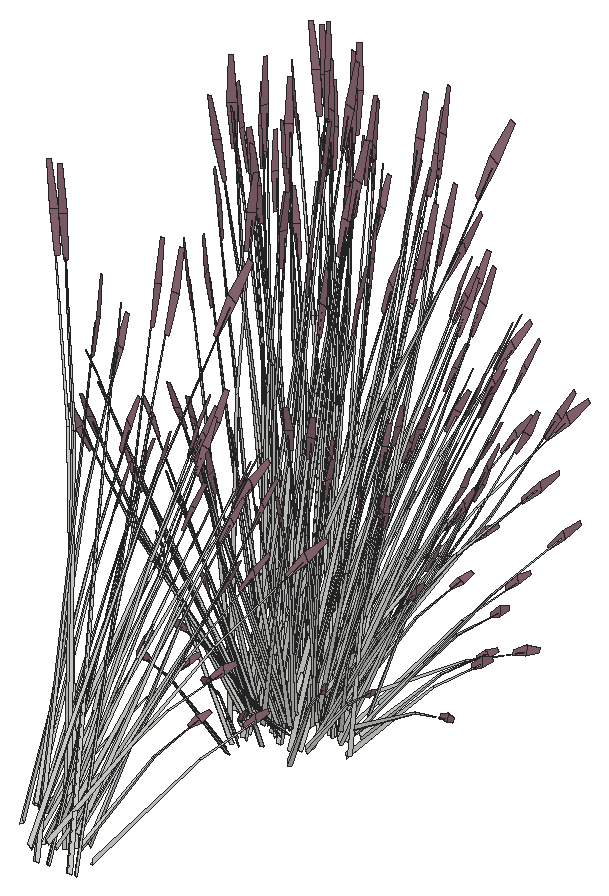
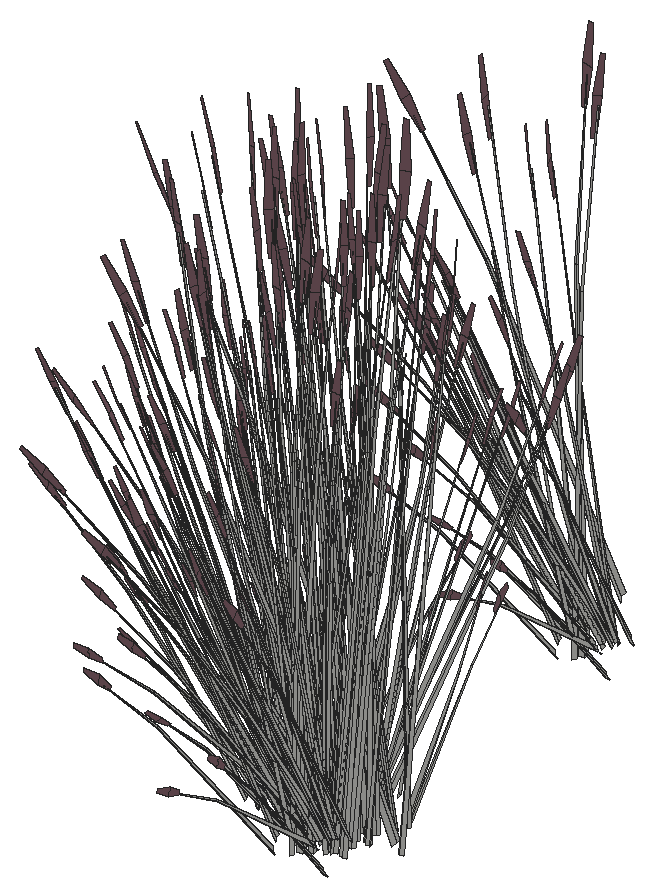
# SketchUp Ruby script. Lengths in inches.
U = 1.inch
M = Sketchup.active_model
def pt(a) = Geom::Point3d.new(a.map { |v| v * U })
def face(e, loops, mat)
  f = e.add_face(loops[0].map { |a| pt(a) })
  loops[1..].each { |l| e.add_face(l.map { |a| pt(a) }).erase! }
  f.material = f.back_material = mat if mat
  f
end
# faces: each face lists its corners as indices into pts; further lists are holes
def faces(e, pts, list, mat = nil) = list.each { |f| face(e, (f[0].is_a?(Array) ? f : [f]).map { |l| l.map { |i| pts[i] } }, mat) }
# xy, xz, yz: faces in a plane at the given z, y or x. An outline is a flat list of corners, or four numbers for a rectangle; further outlines are holes
def ring(l) = l.size == 4 ? [[l[0], l[1]], [l[2], l[1]], [l[2], l[3]], [l[0], l[3]]] : l.each_slice(2).to_a
def flat(e, list, mat, &to3) = list.each { |f| face(e, (f[0].is_a?(Array) ? f : [f]).map { |l| ring(l).map { |u, v| to3.(u, v) } }, mat) }
def xy(e, z, list, mat = nil) = flat(e, list, mat) { |x, y| [x, y, z] }
def xz(e, y, list, mat = nil) = flat(e, list, mat) { |x, z| [x, y, z] }
def yz(e, x, list, mat = nil) = flat(e, list, mat) { |y, z| [x, y, z] }
def lines(e, pts, list) = list.each { |a, b| e.add_line(pt(pts[a]), pt(pts[b])) }
# prism: a flat outline (further loops are holes) pulled along v
def prism(e, loops, v, mat = nil)
  f = face(e, loops, mat); d = Geom::Vector3d.new(v.map { |x| x * U })
  f.pushpull(f.normal.samedirection?(d) ? d.length : -d.length)
end
def box(e, o, s, mat = nil) = prism(e, [[o, [o[0] + s[0], o[1], o[2]], [o[0] + s[0], o[1] + s[1], o[2]], [o[0], o[1] + s[1], o[2]]]], [0, 0, s[2]], mat)
def at(x, y, z, deg = 0) = Geom::Transformation.translation(pt([x, y, z])) * Geom::Transformation.rotation(ORIGIN, Z_AXIS, deg.degrees)
def axes(o, x, y, z) = Geom::Transformation.new([*x, 0, *y, 0, *z, 0, *pt(o).to_a, 1])
def part(name) = M.definitions.add(name)
# library, detail: a bought-in or finely detailed component or shape, given as its bounding box
def library(name, o, s) = part(name).tap { |d| box(d.entities, o, s) }
def detail(e, o, s) = box(e.add_group.entities, o, s)
def put(e, d, t, mat = nil) = e.add_instance(d, t).tap { |i| i.material = mat if mat }
def group(e, t, mat = nil) = e.add_group.tap { |g| g.transformation = t; g.material = mat if mat }.entities
root = M.entities
M.materials.add("LightPink_Translucent").color = [144, 107, 117]
c1 = part("blade")
p = [[2.15,0.21,22],[0,0.17,0],[0.09,0.45,0],[2.18,0.31,22],[2.29,0.31,22],[0.38,0.45,0],
  [2.48,0.24,33],[2.49,0.24,33],[2.48,0.22,33]]
faces(c1.entities,p,[[0,1,2,3],[4,5,2,3],[6,3,4,7],[8,0,3,6]])
c2 = part("seeds")
p = [[0.3,-0.1,1.38],[-0.01,-0.03,1.59],[-0.01,-0.03,0.03],[0.14,-0.07,-0.07],[0.29,-0.03,3],[0.15,0.01,3.11]]
faces(c2.entities,p,[[0,1,2,3],[1,0,4,5]],"LightPink_Translucent")
c3 = part("blade with seeds")
put(c3.entities,c1,at(0,0,0))
put(c3.entities,c2,axes([2.4,0.25,30.99],[1.5799,-0.05474,1.17369],[-0.12525,1.92788,0.29478],[-0.07173,-0.02425,1.56792]))
put(root,c3,axes([76.63,462.61,35.41],[-1.19922,0.48218,-0.1216],[-0.58932,-0.85579,-0.67495],[-0.15822,-0.36063,1.02557]))
put(root,c3,axes([75.6,462.65,35.06],[-1.20468,-0.25962,-0.51099],[0.41292,-0.89013,-0.3958],[-0.11046,-0.35838,0.97773]))
put(root,c3,axes([73.38,434.68,36.3],[-0.02999,-0.3975,1.71376],[1.30002,0.26369,0.13857],[-0.08041,0.56647,0.73262]))
put(root,c3,axes([73.38,469.24,34.25],[-0.02999,-0.3975,1.71376],[1.30002,0.26369,0.13857],[-0.08041,0.56647,0.73262]))
put(root,c3,axes([70.95,465.85,32.4],[0.85545,-0.64616,-0.30978],[0.85545,0.64616,0.30978],[0,-0.20813,1.38974]))
put(root,c3,axes([74.82,461.68,32.5],[-0.84686,0.59414,-0.03893],[-0.77596,-0.65071,-0.17649],[-0.05463,-0.18438,0.58215]))
put(root,c3,axes([74.48,467.54,32.74],[1.54892,0.2182,0.45755],[-0.31522,1.23236,0.17955],[-0.22636,-0.119,1.58856]))
put(root,c3,axes([74.08,467.3125,33.09],[-0.59459,0.93321,0.44739],[-1.23546,-0.44912,-0.21531],[0,-0.21512,1.43643]))
put(root,c3,axes([76.04,462.82,35.36],[-0.5849,-0.8421,-0.71045],[1.20401,-0.4693,0.08574],[-0.13677,-0.40688,1.00501]))
put(root,c3,axes([73.65,469.5,32.85],[1.31687,-0.27488,0.17642],[0.32517,1.02297,0.35086],[-0.11745,-0.14905,1.60407]))
put(root,c3,axes([75.34,469.67,32.57],[-1.23546,-0.46496,0],[0.59459,-0.96613,0],[0,0,1.62707]))
put(root,c3,axes([76.27,462.94,35.43],[-0.36946,0.79643,0.35414],[-1.07787,-0.23229,-0.4572],[-0.09883,-0.32066,0.87481]))
put(root,c3,axes([78.2,436.27,34.8],[0.7662,1.03778,0],[-1.28187,0.57875,-0.51607],[-0.29196,0.13181,1.63711]))
put(root,c3,axes([78.2,470.83,32.75],[0.7662,1.03778,0],[-1.28187,0.57875,-0.51607],[-0.29196,0.13181,1.63711]))
put(root,c3,axes([74.3,436.71,37.49],[-1.20755,-0.27075,0.53283],[0.41292,-0.89013,0.43934],[0.07257,0.35005,1.10256]))
put(root,c3,axes([74.3,471.28,35.44],[-1.20755,-0.27075,0.53283],[0.41292,-0.89013,0.43934],[0.07257,0.35005,1.10256]))
put(root,c3,axes([73.98,436.78,37.16],[-0.90301,0.35198,0.0643],[-0.44199,-0.64184,0.50621],[0.08721,0.28293,0.77189]))
put(root,c3,axes([73.98,471.35,35.11],[-0.90301,0.35198,0.0643],[-0.44199,-0.64184,0.50621],[0.08721,0.28293,0.77189]))
put(root,c3,axes([77.5625,469.5625,32.85],[0.35402,-1.02926,0.17642],[1.29548,0.29127,0.35086],[-0.22379,0.00501,1.60407]))
put(root,c3,axes([76.97,468.2,32.99],[0.90538,0.62224,0.1448],[-0.75521,0.70202,-0.41347],[-0.21021,0.09491,1.26744]))
put(root,c3,axes([76.64,467.43,32.67],[-1.1399,-0.8914,-0.06131],[1.1406,-0.89194,0],[-0.03981,-0.03113,1.75571]))
put(root,c3,axes([76.94,467.74,33.09],[1.33077,-0.06393,0.44739],[0.12035,1.06125,-0.21531],[-0.23824,0.10756,1.43643]))
put(root,c3,axes([77.27,435.61,34.76],[1.53422,0.33662,0.30756],[-0.38383,1.20322,-0.36492],[-0.25393,0.15059,1.64885]))
put(root,c3,axes([77.27,470.18,32.71],[1.53422,0.33662,0.30756],[-0.38383,1.20322,-0.36492],[-0.25393,0.15059,1.64885]))
put(root,c3,axes([75.03,460.95,31.87],[-0.20555,0.03731,1.76342],[-1.13672,-0.42002,-0.26939],[0.01907,-0.35034,0.30037]))
put(root,c3,axes([77.93,470.11,32.85],[1.14694,-0.51783,0.49651],[0.68554,0.92854,0],[-0.26122,0.11794,1.57504]))
put(root,c3,axes([76.15,462.1,34.9],[0.36946,-0.79643,-0.35414],[1.07787,0.23229,0.4572],[-0.09883,-0.32066,0.87481]))
put(root,c3,axes([74.34,466.4,32.74],[0.53281,1.15808,0.45755],[-1.52239,0.4027,0.17955],[0.01861,-0.2128,1.58856]))
put(root,c3,axes([74.1,466.25,32.59],[0.59459,-0.93321,-0.44739],[1.23546,0.44912,0.21531],[0,-0.21512,1.43643]))
put(root,c3,axes([75.62,469.26,32.58],[-0.39985,-0.89288,0],[1.1418,-0.31268,0],[0,0,1.54371]))
put(root,c3,axes([74.17,436.58,33.92],[0.19833,-0.05635,1.76342],[1.19302,0.31018,-0.26939],[0.03489,0.3496,0.30037]))
put(root,c3,axes([74.17,471.15,31.87],[0.19833,-0.05635,1.76342],[1.19302,0.31018,-0.26939],[0.03489,0.3496,0.30037]))
put(root,c3,axes([74.43,436.9,36.95],[-0.36946,0.79643,-0.35414],[-1.07787,-0.23229,0.4572],[0.09883,0.32066,0.87481]))
put(root,c3,axes([74.43,471.46,34.9],[-0.36946,0.79643,-0.35414],[-1.07787,-0.23229,0.4572],[0.09883,0.32066,0.87481]))
put(root,c3,axes([77.24,432.9375,34.64],[-0.59459,0.93321,-0.44739],[-1.23546,-0.44912,0.21531],[0,0.21512,1.43643]))
put(root,c3,axes([77.24,467.5,32.59],[-0.59459,0.93321,-0.44739],[-1.23546,-0.44912,0.21531],[0,0.21512,1.43643]))
put(root,c3,axes([76.6,462.22,35.11],[0.90301,-0.35198,0.0643],[0.44199,0.64184,0.50621],[-0.08721,-0.28293,0.77189]))
put(root,c3,axes([73.67,438.31,37.14],[0.15534,0.16677,1.74944],[1.25362,0.06552,-0.27667],[0.12606,0.3678,0.14031]))
put(root,c3,axes([73.67,472.875,35.09],[0.15534,0.16677,1.74944],[1.25362,0.06552,-0.27667],[0.12606,0.3678,0.14031]))
put(root,c3,axes([79.59,466.94,32.85],[-0.96285,-0.75439,0.17642],[0.97031,-0.7317,0.35086],[-0.10634,0.15406,1.60407]))
put(root,c3,axes([76.26,466.5,32.58],[0,-1.19833,0],[1.53239,0,0],[0,0,1.79456]))
put(root,c3,axes([76.28,462.29,35.11],[1.20755,0.27075,0.48003],[-0.41292,0.89013,0.3958],[-0.07257,-0.35005,0.9933]))
put(root,c3,axes([74.84,466.72,32.81],[1.3808,0.50196,0.24065],[-0.66454,1.04299,0.50002],[0,-0.24043,1.60543]))
put(root,c3,axes([77.03,466.98,32.67],[0,1.19774,-0.05637],[-1.53239,0,0],[0,0.03764,1.79368]))
put(root,c3,axes([74.39,466.02,33.09],[-1.33077,0.06393,0.44739],[-0.12035,-1.06125,-0.21531],[0.23824,-0.10756,1.43643]))
put(root,c3,axes([74.3125,436.06,37.48],[0.36946,-0.79643,0.35414],[1.07787,0.23229,-0.4572],[0.09883,0.32066,0.87481]))
put(root,c3,axes([74.3125,470.625,35.43],[0.36946,-0.79643,0.35414],[1.07787,0.23229,-0.4572],[0.09883,0.32066,0.87481]))
put(root,c3,axes([73.77,464.2,32.85],[-0.35402,1.02926,0.17642],[-1.29548,-0.29127,0.35086],[0.22379,-0.00501,1.60407]))
put(root,c3,axes([76.3,469.3,32.67],[0.53281,1.18979,-0.06012],[-1.52239,0.41691,0],[0.01861,0.04155,1.72173]))
put(root,c3,axes([73.14,462.93,32.75],[-0.7662,-1.03778,0],[1.28187,-0.57875,-0.51607],[0.29196,-0.13181,1.63711]))
put(root,c3,axes([74.54,436.18,37.41],[0.5849,0.8421,-0.71045],[-1.20401,0.4693,0.08574],[0.13677,0.40688,1.00501]))
put(root,c3,axes([74.54,470.75,35.36],[0.5849,0.8421,-0.71045],[-1.20401,0.4693,0.08574],[0.13677,0.40688,1.00501]))
put(root,c3,axes([80.7,467.73,32.58],[-1.53164,-0.00828,-0.04976],[0,-1.1575,0.49943],[-0.04813,0.2635,1.58352]))
put(root,c3,axes([77.6875,464.25,32.85],[-1.31687,0.27488,0.17642],[-0.32517,-1.02297,0.35086],[0.11745,0.14905,1.60407]))
put(root,c3,axes([76.34,460.42,33.14],[0.15721,0.60392,1.1486],[-0.87211,-0.33448,0.84392],[0.09385,-0.30923,0.25299]))
put(root,c3,axes([75.76,438.9,38.07],[0.84686,-0.59414,-0.06488],[0.77596,0.65071,-0.29416],[0.05463,0.18438,0.97024]))
put(root,c3,axes([75.76,473.47,36.02],[0.84686,-0.59414,-0.06488],[0.77596,0.65071,-0.29416],[0.05463,0.18438,0.97024]))
put(root,c3,axes([75.53,465.74,32.74],[-1.01611,0.93987,0.45755],[-1.20717,-0.82966,0.17955],[0.24496,-0.0938,1.58856]))
put(root,c3,axes([77.27,467.23,32.59],[0.85545,0.66896,0],[-0.85545,0.66896,0],[0,0,1.69266]))
put(root,c3,axes([77.26,466.44,33.09],[0.59459,-0.93321,0.44739],[1.23546,0.44912,-0.21531],[0,0.21512,1.43643]))
put(root,c3,axes([76.74,469.69,32.58],[1.23546,0.46496,0],[-0.59459,0.96613,0],[0,0,1.74954]))
put(root,c3,axes([74.98,436.35,37.11],[1.20468,0.25962,-0.51099],[-0.41292,0.89013,-0.3958],[0.11046,0.35838,0.97773]))
put(root,c3,axes([74.98,470.92,35.06],[1.20468,0.25962,-0.51099],[-0.41292,0.89013,-0.3958],[0.11046,0.35838,0.97773]))
put(root,c3,axes([73.95,436.39,37.46],[1.19922,-0.48218,-0.1216],[0.58932,0.85579,-0.67495],[0.15822,0.36063,1.02557]))
put(root,c3,axes([73.95,470.96,35.41],[1.19922,-0.48218,-0.1216],[0.58932,0.85579,-0.67495],[0.15822,0.36063,1.02557]))
put(root,c3,axes([76.86,466.22,32.76],[-1.54892,-0.2182,0.49198],[0.31522,-1.23236,0.19306],[0.22636,0.119,1.70813]))
put(root,c3,axes([80.08,461.4,35.08],[-0.12446,0.07911,1.77383],[-1.21937,-0.26689,-0.16761],[-0.04414,-0.34521,0.31391]))
put(root,c3,axes([79.12,463.6875,35.41],[-1.34686,-0.05131,-0.1216],[0.03681,-0.97156,-0.67495],[0.09356,-0.37418,1.02557]))
put(root,c3,axes([80.38,433.34,34.46],[-0.85545,0.64616,-0.30978],[-0.85545,-0.64616,0.30978],[0,0.20813,1.38974]))
put(root,c3,axes([80.38,467.9,32.4],[-0.85545,0.64616,-0.30978],[-0.85545,-0.64616,0.30978],[0,0.20813,1.38974]))
put(root,c3,axes([77.94,433.22,34.52],[0.44936,0.94823,-0.69212],[-1.29441,0.3415,-0.18165],[0.04967,0.32109,1.52773]))
put(root,c3,axes([77.94,467.78,32.47],[0.44936,0.94823,-0.69212],[-1.29441,0.3415,-0.18165],[0.04967,0.32109,1.52773]))
put(root,c3,axes([77.3,466.77,32.58],[1.37109,0,0],[0,1.07219,0],[0,0,1.78407]))
put(root,c3,axes([78.59,463.84,35.43],[-0.82919,0.54528,0.35414],[-0.78493,-0.62262,-0.4572],[0.11943,-0.31634,0.87481]))
put(root,c3,axes([75.98,465.58,33.09],[-0.73619,-0.86927,0.44739],[1.11511,-0.61213,-0.21531],[0.23824,0.10756,1.43643]))
put(root,c3,axes([74.64,465.79,33.04],[-0.1428,-1.18174,-0.29095],[1.48733,-0.07145,-0.50002],[0.26191,-0.15741,1.59708]))
put(root,c3,axes([77.77,466.66,32.99],[1.1418,-0.30203,0.1448],[0.39985,0.86246,-0.41347],[0,0.18981,1.26744]))
put(root,c3,axes([78.2,463.32,35.06],[-0.87728,-0.69587,-0.51099],[0.92674,-0.60943,-0.3958],[0.13348,-0.35356,0.97773]))
put(root,c3,axes([77.38,466.73,33.04],[1.38012,0.49416,-0.29095],[-0.66454,1.04299,-0.50002],[0.04337,0.25608,1.59708]))
put(root,c3,axes([74.45,463.18,32.4],[1.14332,0.25625,-0.30978],[-0.28787,0.90242,0.30978],[0.23049,-0.10406,1.38974]))
put(root,c3,axes([77.625,462.09,32.97],[-0.34835,0.20963,1.43002],[-1.04325,-0.36691,-0.30754],[0.19338,-0.4563,0.61141]))
put(root,c3,axes([80.38,466.96,32.85],[0,-1.03566,0.49651],[1.37109,0,0],[0,0.23588,1.57504]))
put(root,c3,axes([80.97,433.36,34.45],[0,1.03566,-0.49651],[-1.37109,0,0],[0,0.23588,1.57504]))
put(root,c3,axes([80.97,467.93,32.39],[0,1.03566,-0.49651],[-1.37109,0,0],[0,0.23588,1.57504]))
put(root,c3,axes([77.31,436.5,37.16],[-1.21888,0.23767,0.48003],[-0.21154,-0.93233,0.3958],[0.28666,0.27478,0.9933]))
put(root,c3,axes([77.31,471.0625,35.11],[-1.21888,0.23767,0.48003],[-0.21154,-0.93233,0.3958],[0.28666,0.27478,0.9933]))
put(root,c3,axes([74.18,462.77,32.39],[1.14694,-0.51783,-0.49651],[0.68554,0.92854,0],[0.26122,-0.11794,1.57504]))
put(root,c3,axes([77.07,436.68,37.16],[-0.55698,0.6579,0.0643],[-0.79316,-0.38303,0.50621],[0.25643,0.21093,0.77189]))
put(root,c3,axes([77.07,471.25,35.11],[-0.55698,0.6579,0.0643],[-0.79316,-0.38303,0.50621],[0.25643,0.21093,0.77189]))
put(root,c3,axes([75.66,434.51,36.3],[-0.28013,-0.33252,1.71376],[1.29445,-0.27994,0.13857],[0.29256,0.52202,0.73262]))
put(root,c3,axes([75.66,469.08,34.25],[-0.28013,-0.33252,1.71376],[1.29445,-0.27994,0.13857],[0.29256,0.52202,0.73262]))
put(root,c3,axes([76.48,465.34,32.99],[0.23642,-0.92427,0.1448],[1.15506,0.16044,-0.41347],[0.21021,0.09491,1.26744]))
put(root,c3,axes([78.12,463.73,32.85],[-1.14694,-0.51783,0.49651],[0.68554,-0.92854,0],[0.26122,0.11794,1.57504]))
put(root,c3,axes([78.47,463.64,35.36],[0.03189,-0.95798,-0.71045],[1.34277,0.06434,0.08574],[0.14171,-0.40585,1.00501]))
put(root,c3,axes([77.12,469.14,32.5625],[1.2866,-0.3514,-0.19198],[0.45209,1.01223,0.00008],[0.14202,-0.03884,1.73897]))
put(root,c3,axes([76.9,435.93,37.48],[-0.18927,-0.83419,0.35414],[1.08199,-0.22027,-0.4572],[0.29062,0.23905,0.87481]))
put(root,c3,axes([76.9,470.49,35.43],[-0.18927,-0.83419,0.35414],[1.08199,-0.22027,-0.4572],[0.29062,0.23905,0.87481]))
put(root,c3,axes([77.14,466.13,32.59],[0.73619,0.86927,-0.44739],[-1.11511,0.61213,0.21531],[0.23824,0.10756,1.43643]))
put(root,c3,axes([77.63,431.13,36.9],[-1.05895,-0.53811,1.38283],[1.11816,-0.83781,0.59665],[0.34166,0.5049,1.33663]))
put(root,c3,axes([77.63,465.69,34.85],[-1.05895,-0.53811,1.38283],[1.11816,-0.83781,0.59665],[0.34166,0.5049,1.33663]))
put(root,c3,axes([79.03,463.06,34.9],[0.82919,-0.54528,-0.35414],[0.78493,0.62262,0.4572],[0.11943,-0.31634,0.87481]))
put(root,c3,axes([75.85,437.09,37.14],[0.00363,-0.12539,1.77383],[1.0502,-0.55319,-0.16761],[0.36479,0.19745,0.31391]))
put(root,c3,axes([75.85,471.66,35.08],[0.00363,-0.12539,1.77383],[1.0502,-0.55319,-0.16761],[0.36479,0.19745,0.31391]))
put(root,c3,axes([79.35,463.34,35.11],[1.00708,0.04826,0.0643],[-0.02761,0.72867,0.50621],[0.10538,-0.27912,0.77189]))
put(root,c3,axes([79.23,435.51,35.19],[-0.69001,-0.29779,1.1486],[0.89096,-0.30257,0.84392],[0.24031,0.2563,0.25299]))
put(root,c3,axes([79.23,470.07,33.14],[-0.69001,-0.29779,1.1486],[0.89096,-0.30257,0.84392],[0.24031,0.2563,0.25299]))
put(root,c3,axes([76.77,435.19,35.02],[0.02163,-0.34331,1.43002],[1.03345,-0.38348,-0.30754],[0.31903,0.4109,0.61141]))
put(root,c3,axes([76.77,469.76,32.97],[0.02163,-0.34331,1.43002],[1.03345,-0.38348,-0.30754],[0.31903,0.4109,0.61141]))
put(root,c3,axes([80.35,462.14,35.09],[-0.01183,-0.20612,1.74944],[-0.99913,-0.59572,-0.27667],[0.15447,-0.36112,0.14031]))
put(root,c3,axes([75.54,464.89,32.44],[0.82544,-0.77843,-0.62353],[1.0254,0.70586,-0.16365],[0.33076,-0.19418,1.37633]))
put(root,c3,axes([79.02,463.28,35.11],[0.87265,0.70663,0.48003],[-0.92674,0.60943,0.3958],[0.16097,-0.33153,0.9933]))
put(root,c3,axes([79.16,464.2,32.4],[0.28787,0.90242,-0.30978],[-1.14332,0.25625,0.30978],[0.23049,0.10406,1.38974]))
put(root,c3,axes([81.31,467.14,32.75],[1.53239,0,0],[0,1.1575,-0.51607],[0,0.26363,1.63711]))
put(root,c3,axes([76.36,465.64,33.04],[1.23732,-0.68758,-0.29095],[0.8228,0.97154,-0.50002],[0.30528,0.09867,1.59708]))
put(root,c3,axes([79.34,436.86,35.1],[-0.78586,-0.03248,1.0506],[0.51898,-0.68985,0.58006],[0.31045,0.24509,0.8241]))
put(root,c3,axes([79.34,471.43,33.04],[-0.78586,-0.03248,1.0506],[0.51898,-0.68985,0.58006],[0.31045,0.24509,0.8241]))
put(root,c3,axes([80.03,465.52,35.43],[-1.06674,0.14801,0.35414],[-0.28168,-0.84611,-0.4572],[0.30569,-0.22726,0.87481]))
put(root,c3,axes([76.96,463.15,34.25],[-0.22818,0.35597,1.71376],[-0.95725,-0.73667,0.13857],[0.43183,-0.45914,0.73262]))
put(root,c3,axes([76.8,436.36,37.46],[0.73026,-0.88648,-0.1216],[1.05755,0.51071,-0.67495],[0.36761,0.25045,1.02557]))
put(root,c3,axes([76.8,470.92,35.41],[0.73026,-0.88648,-0.1216],[1.05755,0.51071,-0.67495],[0.36761,0.25045,1.02557]))
put(root,c3,axes([73.23,465.03,31.97],[-1.20625,0.41464,1.28929],[-0.38394,-1.1897,0.50096],[0.74071,0.01979,1.46642]))
put(root,c3,axes([80.59,465.6,35.41],[-1.1336,-0.57106,-0.1216],[0.65308,-0.827,-0.67495],[0.32027,-0.28747,1.02557]))
put(root,c3,axes([77.67,435.92,37.11],[1.20928,-0.24619,-0.51099],[0.21154,0.93233,-0.3958],[0.32481,0.26718,0.97773]))
put(root,c3,axes([77.67,470.48,35.06],[1.20928,-0.24619,-0.51099],[0.21154,0.93233,-0.3958],[0.32481,0.26718,0.97773]))
put(root,c3,axes([78.78,463.1875,32.75],[0.7662,-1.03778,0],[1.28187,0.57875,-0.51607],[0.29196,0.13181,1.63711]))
put(root,c3,axes([80.0625,462.73,31.87],[-0.18342,-0.08159,1.76342],[-0.47115,-0.9115,-0.26939],[0.31784,-0.24736,0.30037]))
put(root,c3,axes([79.06,469.37,35.43],[-0.69728,-0.64842,0.35414],[0.79619,-0.61382,-0.4572],[0.40453,0.09339,0.87481]))
put(root,c3,axes([79.48,463.8125,32.39],[1.14694,0.51783,-0.49651],[-0.68554,0.92854,0],[0.26122,0.11794,1.57504]))
put(root,c3,axes([79.6875,435.39,37.16],[-0.06171,0.78753,0.0643],[-0.9318,-0.02159,0.50621],[0.35694,0.08241,0.77189]))
put(root,c3,axes([79.6875,469.95,35.11],[-0.06171,0.78753,0.0643],[-0.9318,-0.02159,0.50621],[0.35694,0.08241,0.77189]))
put(root,c3,axes([79.42,436.62,33.92],[0.08928,-0.14952,1.76342],[1.12407,-0.44035,-0.26939],[0.34078,0.22791,0.30037]))
put(root,c3,axes([79.42,471.18,31.87],[0.08928,-0.14952,1.76342],[1.12407,-0.44035,-0.26939],[0.34078,0.22791,0.30037]))
put(root,c3,axes([79.77,435.14,37.16],[-0.90362,0.68241,0.48003],[-0.77932,-0.72471,0.3958],[0.42395,0.12588,0.9933]))
put(root,c3,axes([79.77,469.7,35.11],[-0.90362,0.68241,0.48003],[-0.77932,-0.72471,0.3958],[0.42395,0.12588,0.9933]))
put(root,c3,axes([80.02,464.92,35.06],[-0.31482,-0.94565,-0.51099],[1.19224,-0.16542,-0.3958],[0.34166,-0.254,0.97773]))
put(root,c3,axes([82.12,469.8,34.31],[-0.23455,-0.87059,-0.03492],[1.10861,-0.20015,-0.15832],[0.23151,0.05519,0.52218]))
put(root,c3,axes([80.2,467.55,35.43],[-1.01846,-0.28891,0.35414],[0.29705,-0.84289,-0.4572],[0.41005,-0.07729,0.87481]))
put(root,c3,axes([77.8,465.8,32.44],[1.27479,0.1698,-0.62353],[-0.26901,1.04736,-0.16365],[0.38043,0.12691,1.37633]))
put(root,c3,axes([83.23,466.41,32.64],[-0.75977,-0.66224,-0.06488],[0.83212,-0.6068,-0.29416],[0.23578,-0.04272,0.97024]))
put(root,c3,axes([81.49,463.04,33.14],[-0.40819,0.5272,1.1486],[-0.35086,-0.70831,0.84392],[0.33713,-0.17749,0.25299]))
put(root,c3,axes([81,465.39,35.11],[0.8413,0.43556,0.0643],[-0.48981,0.62025,0.50621],[0.26973,-0.20053,0.77189]))
put(root,c3,axes([80.77,465.21,35.11],[0.30393,0.95317,0.48003],[-1.19224,0.16542,0.3958],[0.35138,-0.22417,0.9933]))
put(root,c3,axes([77.54,433.48,36.3],[-0.45521,-0.17844,1.71376],[0.94204,-0.74856,0.13857],[0.58713,0.33769,0.73262]))
put(root,c3,axes([77.54,468.04,34.25],[-0.45521,-0.17844,1.71376],[0.94204,-0.74856,0.13857],[0.58713,0.33769,0.73262]))
put(root,c3,axes([83.38,465.35,35.08],[-0.16006,-0.00787,1.77383],[-0.66468,-0.8428,-0.16761],[0.26693,-0.27711,0.31391]))
put(root,c3,axes([80.9,465.02,34.9],[1.06674,-0.14801,-0.35414],[0.28168,0.84611,0.4572],[0.30569,-0.22726,0.87481]))
put(root,c3,axes([80.06,465.31,35.36],[0.64013,-0.81717,-0.71045],[1.12174,0.58074,0.08574],[0.38221,-0.29607,1.00501]))
put(root,c3,axes([81.125,467.81,35.11],[0.4501,0.70615,0.0643],[-0.82077,0.34564,0.50621],[0.36181,-0.0682,0.77189]))
put(root,c3,axes([80.05,469.7,34.9],[0.69728,0.64842,-0.35414],[-0.79619,0.61382,0.4572],[0.40453,0.09339,0.87481]))
put(root,c3,axes([79.25,469.78,35.41],[0.06562,-1.05324,-0.1216],[1.2424,0.02879,-0.67495],[0.4785,0.07316,1.02557]))
put(root,c3,axes([80.63,467.83,35.41],[-0.6166,-0.93779,-0.1216],[1.09436,-0.46085,-0.67495],[0.46117,-0.12373,1.02557]))
put(root,c3,axes([81.04,467.56,35.11],[-0.34623,0.9443,0.48003],[-1.13828,-0.3229,0.3958],[0.44763,-0.05675,0.9933]))
put(root,c3,axes([80.33,469.15,35.09],[0.26289,-0.01751,1.74944],[0.72108,-0.8046,-0.27667],[0.46761,0.10621,0.14031]))
put(root,c3,axes([80.58,467.02,35.06],[0.332,-0.94205,-0.51099],[1.13828,0.3229,-0.3958],[0.45829,-0.08638,0.97773]))
put(root,c3,axes([83.4375,467.625,33.14],[-0.75718,0.17097,1.1486],[0.35641,-0.70661,0.84392],[0.40168,0.04835,0.25299]))
put(root,c3,axes([80.98,464.56,32.97],[-0.4378,-0.03068,1.43002],[-0.44851,-0.8229,-0.30754],[0.53783,-0.23279,0.61141]))
put(root,c3,axes([81.28,467.45,34.9],[1.01846,0.28891,-0.35414],[-0.29705,0.84289,0.4572],[0.41005,-0.07729,0.87481]))
put(root,c3,axes([79.31,469.27,35.36],[1.22504,0.02494,-0.71045],[-0.08228,1.05005,0.08574],[0.51899,0.11081,1.00501]))
put(root,c3,axes([81.79,467.29,32.36],[-0.7893,0.12429,1.41583],[-0.12563,-0.9893,0.08104],[0.55282,-0.14974,0.80566]))
put(root,c3,axes([82.66,466.64,31.87],[-0.06405,-0.15723,1.76342],[0.44421,-0.91974,-0.26939],[0.4481,-0.01323,0.30037]))
put(root,c3,axes([83.08,470.62,35.08],[-0.11081,-0.09067,1.77383],[0.2424,-0.97188,-0.16761],[0.43649,-0.06209,0.31391]))
put(root,c3,axes([78.5,466.41,34.25],[-0.50831,0.02346,1.71376],[0.33721,-1.01661,0.13857],[0.72439,0.06288,0.73262]))
put(root,c3,axes([80.36,467.37,35.36],[1.07686,-0.45739,-0.71045],[0.60013,0.94154,0.08574],[0.52031,-0.10696,1.00501]))
put(root,c3,axes([83.98,466.36,35.09],[0.17006,-0.15775,1.74944],[-0.21766,-0.96766,-0.27667],[0.42669,-0.18347,0.14031]))
put(root,c3,axes([82.02,468.76,32.97],[-0.29514,-0.25472,1.43002],[0.38401,-0.84262,-0.30754],[0.59714,0.11414,0.61141]))
